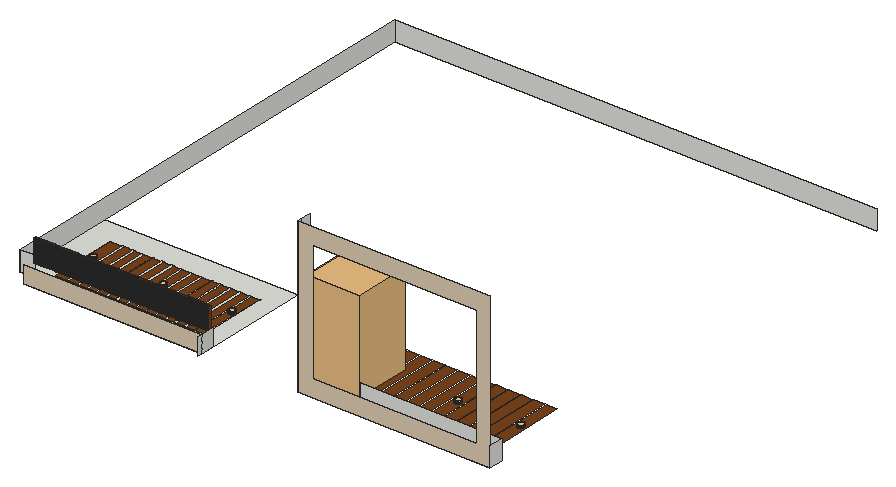
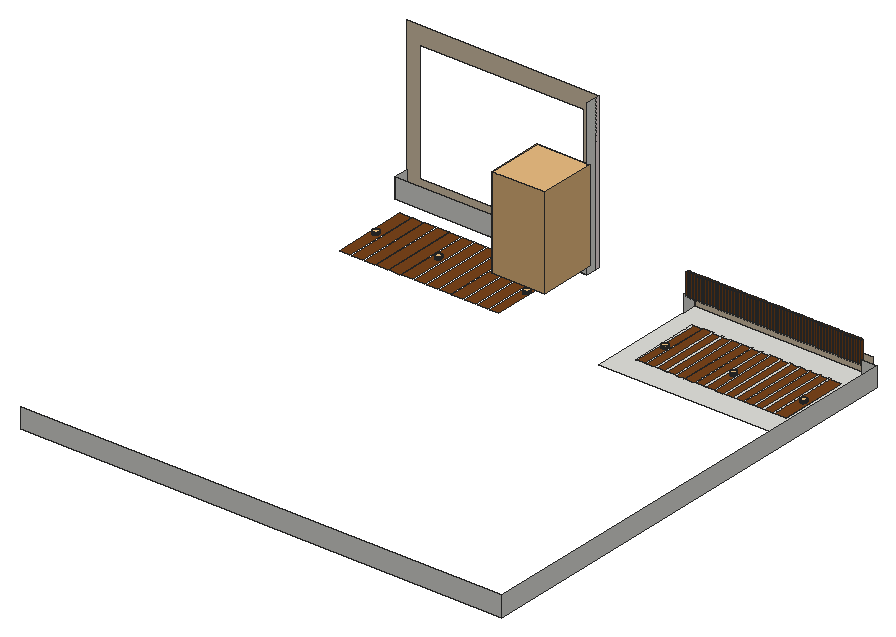
# SketchUp Ruby script. Lengths in inches.
U = 1.inch
M = Sketchup.active_model
def pt(a) = Geom::Point3d.new(a.map { |v| v * U })
def face(e, loops, mat)
  f = e.add_face(loops[0].map { |a| pt(a) })
  loops[1..].each { |l| e.add_face(l.map { |a| pt(a) }).erase! }
  f.material = f.back_material = mat if mat
  f
end
# faces: each face lists its corners as indices into pts; further lists are holes
def faces(e, pts, list, mat = nil) = list.each { |f| face(e, (f[0].is_a?(Array) ? f : [f]).map { |l| l.map { |i| pts[i] } }, mat) }
# xy, xz, yz: faces in a plane at the given z, y or x. An outline is a flat list of corners, or four numbers for a rectangle; further outlines are holes
def ring(l) = l.size == 4 ? [[l[0], l[1]], [l[2], l[1]], [l[2], l[3]], [l[0], l[3]]] : l.each_slice(2).to_a
def flat(e, list, mat, &to3) = list.each { |f| face(e, (f[0].is_a?(Array) ? f : [f]).map { |l| ring(l).map { |u, v| to3.(u, v) } }, mat) }
def xy(e, z, list, mat = nil) = flat(e, list, mat) { |x, y| [x, y, z] }
def xz(e, y, list, mat = nil) = flat(e, list, mat) { |x, z| [x, y, z] }
def yz(e, x, list, mat = nil) = flat(e, list, mat) { |y, z| [x, y, z] }
def lines(e, pts, list) = list.each { |a, b| e.add_line(pt(pts[a]), pt(pts[b])) }
# prism: a flat outline (further loops are holes) pulled along v
def prism(e, loops, v, mat = nil)
  f = face(e, loops, mat); d = Geom::Vector3d.new(v.map { |x| x * U })
  f.pushpull(f.normal.samedirection?(d) ? d.length : -d.length)
end
def box(e, o, s, mat = nil) = prism(e, [[o, [o[0] + s[0], o[1], o[2]], [o[0] + s[0], o[1] + s[1], o[2]], [o[0], o[1] + s[1], o[2]]]], [0, 0, s[2]], mat)
def at(x, y, z, deg = 0) = Geom::Transformation.translation(pt([x, y, z])) * Geom::Transformation.rotation(ORIGIN, Z_AXIS, deg.degrees)
def axes(o, x, y, z) = Geom::Transformation.new([*x, 0, *y, 0, *z, 0, *pt(o).to_a, 1])
def part(name) = M.definitions.add(name)
# library, detail: a bought-in or finely detailed component or shape, given as its bounding box
def library(name, o, s) = part(name).tap { |d| box(d.entities, o, s) }
def detail(e, o, s) = box(e.add_group.entities, o, s)
def put(e, d, t, mat = nil) = e.add_instance(d, t).tap { |i| i.material = mat if mat }
def group(e, t, mat = nil) = e.add_group.tap { |g| g.transformation = t; g.material = mat if mat }.entities
root = M.entities
M.materials.add("Generic\#1").color = [121, 68, 27]
M.materials.add("Generic\#2").color = [245, 199, 133]
M.materials.add("Generic\#6").color = [223, 205, 179]
M.materials.add("Generic\#9").color = [246, 231, 231]
c1 = library("Plante 4",[-1.67,-6.5,0],[37.31,31.95,64.42])
c2 = part("Group\#9")
xy(c2.entities,22.76,[[0,0,2,3]])
xz(c2.entities,0,[[0,0,2,22.76]])
yz(c2.entities,0,[[0,0,3,22.76]])
yz(c2.entities,2,[[0,0,3,22.76]])
xy(root,260.875,[[306.09,39.375,507.875,54.5625],[[17.125,41,204.09,41,204.09,166.1875,2.3125,166.1875,2.3125,54.5625,17.125,54.5625],[27.64,66.32,186.39,140.86]],[40.89,66.32,42.89,140.86],[51.14,66.32,53.14,140.86],[61.39,66.32,63.39,140.86],
  [71.64,66.32,73.64,140.86],[81.89,66.32,83.89,140.86],[92.14,66.32,94.14,140.86],[102.39,66.32,104.39,140.86],[112.64,66.32,114.64,140.86],
  [122.89,66.32,124.89,140.86],[133.14,66.32,135.14,140.86],[143.39,66.32,145.39,140.86],[153.64,66.32,155.64,140.86],[163.89,66.32,165.89,140.86],
  [174.14,66.32,176.14,140.86],[184.39,66.32,186.39,140.86]])
xy(root,260.875,[[[28.83,66.32,40.89,140.86],[34.54,106.62,35.35,106.72,36.11,107.04,36.75,107.53,37.25,108.18,37.5625,108.93,37.67,109.74,37.5625,110.55,37.25,111.3,36.75,111.95,36.11,112.45,35.35,112.76,34.54,112.87,33.74,112.76,32.98,112.45,32.33,111.95,31.84,111.3,31.53,110.55,31.42,109.74,31.53,108.93,31.84,108.18,32.33,107.53,32.98,107.04,33.74,106.72]],[42.89,66.32,51.14,140.86],[53.14,66.32,61.39,140.86],[63.39,66.32,71.64,140.86],[73.64,66.32,81.89,140.86],
  [83.89,66.32,92.14,140.86],[94.14,66.32,102.39,140.86],[[104.39,66.32,112.64,140.86],[108.29,106.62,109.1,106.72,109.86,107.04,110.5,107.53,111,108.18,111.3125,108.93,111.42,109.74,111.3125,110.55,111,111.3,110.5,111.95,109.86,112.45,109.1,112.76,108.29,112.87,107.49,112.76,106.73,112.45,106.08,111.95,105.59,111.3,105.28,110.55,105.17,109.74,105.28,108.93,105.59,108.18,106.08,107.53,106.73,107.04,107.49,106.72]],[114.64,66.32,122.89,140.86],[124.89,66.32,133.14,140.86],
  [135.14,66.32,143.39,140.86],[145.39,66.32,153.64,140.86],[155.64,66.32,163.89,140.86],[165.89,66.32,174.14,140.86],[[176.14,66.32,184.39,140.86],[180.36,106.62,181.17,106.72,181.92,107.04,182.57,107.53,183.0625,108.18,183.375,108.93,183.48,109.74,183.375,110.55,183.0625,111.3,182.57,111.95,181.92,112.45,181.17,112.76,180.36,112.87,179.55,112.76,178.79,112.45,178.15,111.95,177.65,111.3,177.34,110.55,177.23,109.74,177.34,108.93,177.65,108.18,178.15,107.53,178.79,107.04,179.55,106.72]],
  [[322.02,70.49,331.7,150.26],[326.125,105.74,326.97,105.8,327.77,106.08,328.48,106.55,329.03,107.1875,329.41,107.95,329.57,108.78,329.51,109.63,329.24,110.43,328.76,111.14,328.125,111.69,327.36,112.07,326.53,112.23,325.68,112.17,324.88,111.9,324.18,111.42,323.62,110.78,323.25,110.02,323.08,109.1875,323.14,108.34,323.42,107.54,323.89,106.84,324.53,106.28,325.29,105.91]],[333.7,70.49,344.89,150.26],[346.89,70.49,358.07,150.26],[360.07,70.49,371.26,150.26],[373.26,70.49,384.45,150.26],
  [386.45,70.49,397.64,150.26],[399.64,70.49,410.82,150.26],[[412.82,70.49,424.01,150.26],[418.4375,105.74,419.28,105.8,420.08,106.08,420.79,106.55,421.35,107.1875,421.72,107.95,421.88,108.78,421.82,109.63,421.55,110.43,421.08,111.14,420.4375,111.69,419.67,112.07,418.84,112.23,417.99,112.17,417.19,111.9,416.49,111.42,415.93,110.78,415.56,110.02,415.39,109.1875,415.45,108.34,415.73,107.54,416.2,106.84,416.84,106.28,417.6,105.91]],[426.01,70.49,437.2,150.26],[439.2,70.49,450.39,150.26],
  [452.39,70.49,463.57,150.26],[465.57,70.49,476.76,150.26],[[478.76,70.49,489.95,150.26],[484.375,105.74,485.22,105.8,486.02,106.08,486.73,106.55,487.28,107.1875,487.66,107.95,487.82,108.78,487.76,109.63,487.49,110.43,487.01,111.14,486.375,111.69,485.61,112.07,484.78,112.23,483.93,112.17,483.13,111.9,482.43,111.42,481.87,110.78,481.5,110.02,481.33,109.1875,481.39,108.34,481.67,107.54,482.14,106.84,482.78,106.28,483.54,105.91]]],"Generic\#1")
xy(root,263.4375,[[326.125,105.74,325.29,105.91,324.53,106.28,323.89,106.84,323.42,107.54,323.14,108.34,323.08,109.1875,323.25,110.02,323.62,110.78,324.18,111.42,324.88,111.9,325.68,112.17,326.53,112.23,327.36,112.07,328.125,111.69,328.76,111.14,329.24,110.43,329.51,109.63,329.57,108.78,329.41,107.95,329.03,107.1875,328.48,106.55,327.77,106.08,326.97,105.8],[418.4375,105.74,417.6,105.91,416.84,106.28,416.2,106.84,415.73,107.54,415.45,108.34,415.39,109.1875,415.56,110.02,415.93,110.78,416.49,111.42,417.19,111.9,417.99,112.17,418.84,112.23,419.67,112.07,420.4375,111.69,421.08,111.14,421.55,110.43,421.82,109.63,421.88,108.78,421.72,107.95,421.35,107.1875,420.79,106.55,420.08,106.08,419.28,105.8],[484.375,105.74,483.54,105.91,482.78,106.28,482.14,106.84,481.67,107.54,481.39,108.34,481.33,109.1875,481.5,110.02,481.87,110.78,482.43,111.42,483.13,111.9,483.93,112.17,484.78,112.23,485.61,112.07,486.375,111.69,487.01,111.14,487.49,110.43,487.76,109.63,487.82,108.78,487.66,107.95,487.28,107.1875,486.73,106.55,486.02,106.08,485.22,105.8],[34.54,106.62,33.74,106.72,32.98,107.04,32.33,107.53,31.84,108.18,31.53,108.93,31.42,109.74,31.53,110.55,31.84,111.3,32.33,111.95,32.98,112.45,33.74,112.76,34.54,112.87,35.35,112.76,36.11,112.45,36.75,111.95,37.25,111.3,37.5625,110.55,37.67,109.74,37.5625,108.93,37.25,108.18,36.75,107.53,36.11,107.04,35.35,106.72],[108.29,106.62,107.49,106.72,106.73,107.04,106.08,107.53,105.59,108.18,105.28,108.93,105.17,109.74,105.28,110.55,105.59,111.3,106.08,111.95,106.73,112.45,107.49,112.76,108.29,112.87,109.1,112.76,109.86,112.45,110.5,111.95,111,111.3,111.3125,110.55,111.42,109.74,111.3125,108.93,111,108.18,110.5,107.53,109.86,107.04,109.1,106.72],
  [180.36,106.62,179.55,106.72,178.79,107.04,178.15,107.53,177.65,108.18,177.34,108.93,177.23,109.74,177.34,110.55,177.65,111.3,178.15,111.95,178.79,112.45,179.55,112.76,180.36,112.87,181.17,112.76,181.92,112.45,182.57,111.95,183.0625,111.3,183.375,110.55,183.48,109.74,183.375,108.93,183.0625,108.18,182.57,107.53,181.92,107.04,181.17,106.72]],"Generic\#2")
xz(root,39.375,[[[306.09,260.875,507.875,422.625],[321.31,278.625,494.1875,404.6875]]],"Generic\#6")
xz(root,41,[[17.125,260.875,204.09,278.75]],"Generic\#6")
xz(root,54.5625,[[2.3125,260.875,17.125,281.75],[306.09,260.875,507.875,281.75]])
xz(root,546.8125,[[2.3125,260.875,507.875,281.75]])
yz(root,2.3125,[[54.5625,260.875,546.8125,281.75]])
yz(root,204.09,[[35.5625,260.875,41,278.75],[41,260.875,54.5625,278.75]])
yz(root,306.09,[[43.625,260.875,54.5625,422.625]])
yz(root,306.09,[[39.375,260.875,43.625,422.625]],"Generic\#9")
yz(root,507.875,[[39.375,260.875,54.5625,281.75]])
p = [[326.125,105.74,260.875],[325.29,105.91,260.875],[325.29,105.91,263.4375],[326.125,105.74,263.4375],[326.97,105.8,260.875],[326.97,105.8,263.4375],
  [418.4375,105.74,260.875],[417.6,105.91,260.875],[417.6,105.91,263.4375],[418.4375,105.74,263.4375],[419.28,105.8,260.875],[419.28,105.8,263.4375],
  [484.375,105.74,260.875],[483.54,105.91,260.875],[483.54,105.91,263.4375],[484.375,105.74,263.4375],[485.22,105.8,260.875],[485.22,105.8,263.4375],
  [327.77,106.08,260.875],[327.77,106.08,263.4375],[420.08,106.08,260.875],[420.08,106.08,263.4375],[486.02,106.08,260.875],[486.02,106.08,263.4375],
  [324.53,106.28,260.875],[324.53,106.28,263.4375],[416.84,106.28,260.875],[416.84,106.28,263.4375],[482.78,106.28,260.875],[482.78,106.28,263.4375],
  [328.48,106.55,260.875],[328.48,106.55,263.4375],[420.79,106.55,260.875],[420.79,106.55,263.4375],[486.73,106.55,260.875],[486.73,106.55,263.4375],
  [323.89,106.84,260.875],[323.89,106.84,263.4375],[416.2,106.84,260.875],[416.2,106.84,263.4375],[482.14,106.84,260.875],[482.14,106.84,263.4375],
  [329.03,107.1875,260.875],[329.03,107.1875,263.4375],[421.35,107.1875,260.875],[421.35,107.1875,263.4375],[487.28,107.1875,260.875],[487.28,107.1875,263.4375],
  [34.54,106.62,260.875],[33.74,106.72,260.875],[33.74,106.72,263.4375],[34.54,106.62,263.4375],[35.35,106.72,260.875],[35.35,106.72,263.4375],
  [108.29,106.62,260.875],[107.49,106.72,260.875],[107.49,106.72,263.4375],[108.29,106.62,263.4375],[109.1,106.72,260.875],[109.1,106.72,263.4375],
  [180.36,106.62,260.875],[179.55,106.72,260.875],[179.55,106.72,263.4375],[180.36,106.62,263.4375],[181.17,106.72,260.875],[181.17,106.72,263.4375],
  [32.98,107.04,260.875],[32.98,107.04,263.4375],[36.11,107.04,260.875],[36.11,107.04,263.4375],[106.73,107.04,260.875],[106.73,107.04,263.4375],
  [109.86,107.04,260.875],[109.86,107.04,263.4375],[178.79,107.04,260.875],[178.79,107.04,263.4375],[181.92,107.04,260.875],[181.92,107.04,263.4375],
  [323.42,107.54,260.875],[323.42,107.54,263.4375],[415.73,107.54,260.875],[415.73,107.54,263.4375],[481.67,107.54,260.875],[481.67,107.54,263.4375],
  [32.33,107.53,260.875],[32.33,107.53,263.4375],[36.75,107.53,260.875],[36.75,107.53,263.4375],[106.08,107.53,260.875],[106.08,107.53,263.4375],
  [110.5,107.53,260.875],[110.5,107.53,263.4375],[178.15,107.53,260.875],[178.15,107.53,263.4375],[182.57,107.53,260.875],[182.57,107.53,263.4375],
  [329.41,107.95,260.875],[329.41,107.95,263.4375],[421.72,107.95,260.875],[421.72,107.95,263.4375],[487.66,107.95,260.875],[487.66,107.95,263.4375],
  [31.84,108.18,260.875],[31.84,108.18,263.4375],[37.25,108.18,260.875],[37.25,108.18,263.4375],[105.59,108.18,260.875],[105.59,108.18,263.4375],
  [111,108.18,260.875],[111,108.18,263.4375],[177.65,108.18,260.875],[177.65,108.18,263.4375],[183.0625,108.18,260.875],[183.0625,108.18,263.4375],
  [323.14,108.34,260.875],[323.14,108.34,263.4375],[415.45,108.34,260.875],[415.45,108.34,263.4375],[481.39,108.34,260.875],[481.39,108.34,263.4375],
  [329.57,108.78,260.875],[329.57,108.78,263.4375],[421.88,108.78,260.875],[421.88,108.78,263.4375],[487.82,108.78,260.875],[487.82,108.78,263.4375],
  [31.53,108.93,260.875],[31.53,108.93,263.4375],[37.5625,108.93,260.875],[37.5625,108.93,263.4375],[105.28,108.93,260.875],[105.28,108.93,263.4375],
  [111.3125,108.93,260.875],[111.3125,108.93,263.4375],[177.34,108.93,260.875],[177.34,108.93,263.4375],[183.375,108.93,260.875],[183.375,108.93,263.4375],
  [323.08,109.1875,260.875],[323.08,109.1875,263.4375],[415.39,109.1875,260.875],[415.39,109.1875,263.4375],[481.33,109.1875,260.875],[481.33,109.1875,263.4375],
  [329.51,109.63,260.875],[329.51,109.63,263.4375],[421.82,109.63,260.875],[421.82,109.63,263.4375],[487.76,109.63,260.875],[487.76,109.63,263.4375],
  [31.42,109.74,260.875],[31.42,109.74,263.4375],[37.67,109.74,260.875],[37.67,109.74,263.4375],[105.17,109.74,260.875],[105.17,109.74,263.4375],
  [111.42,109.74,260.875],[111.42,109.74,263.4375],[177.23,109.74,260.875],[177.23,109.74,263.4375],[183.48,109.74,260.875],[183.48,109.74,263.4375],
  [323.25,110.02,260.875],[323.25,110.02,263.4375],[415.56,110.02,260.875],[415.56,110.02,263.4375],[481.5,110.02,260.875],[481.5,110.02,263.4375],
  [329.24,110.43,260.875],[329.24,110.43,263.4375],[421.55,110.43,260.875],[421.55,110.43,263.4375],[487.49,110.43,260.875],[487.49,110.43,263.4375],
  [31.53,110.55,260.875],[31.53,110.55,263.4375],[37.5625,110.55,260.875],[37.5625,110.55,263.4375],[105.28,110.55,260.875],[105.28,110.55,263.4375],
  [111.3125,110.55,260.875],[111.3125,110.55,263.4375],[177.34,110.55,260.875],[177.34,110.55,263.4375],[183.375,110.55,260.875],[183.375,110.55,263.4375],
  [323.62,110.78,260.875],[323.62,110.78,263.4375],[415.93,110.78,260.875],[415.93,110.78,263.4375],[481.87,110.78,260.875],[481.87,110.78,263.4375],
  [328.76,111.14,260.875],[328.76,111.14,263.4375],[421.08,111.14,260.875],[421.08,111.14,263.4375],[487.01,111.14,260.875],[487.01,111.14,263.4375],
  [31.84,111.3,260.875],[31.84,111.3,263.4375],[37.25,111.3,260.875],[37.25,111.3,263.4375],[105.59,111.3,260.875],[105.59,111.3,263.4375],
  [111,111.3,260.875],[111,111.3,263.4375],[177.65,111.3,260.875],[177.65,111.3,263.4375],[183.0625,111.3,260.875],[183.0625,111.3,263.4375],
  [324.18,111.42,260.875],[324.18,111.42,263.4375],[416.49,111.42,260.875],[416.49,111.42,263.4375],[482.43,111.42,260.875],[482.43,111.42,263.4375],
  [328.125,111.69,260.875],[328.125,111.69,263.4375],[420.4375,111.69,260.875],[420.4375,111.69,263.4375],[486.375,111.69,260.875],[486.375,111.69,263.4375],
  [32.33,111.95,260.875],[32.33,111.95,263.4375],[36.75,111.95,260.875],[36.75,111.95,263.4375],[106.08,111.95,260.875],[106.08,111.95,263.4375],
  [110.5,111.95,260.875],[110.5,111.95,263.4375],[178.15,111.95,260.875],[178.15,111.95,263.4375],[182.57,111.95,260.875],[182.57,111.95,263.4375],
  [324.88,111.9,260.875],[324.88,111.9,263.4375],[417.19,111.9,260.875],[417.19,111.9,263.4375],[483.13,111.9,260.875],[483.13,111.9,263.4375],
  [327.36,112.07,260.875],[327.36,112.07,263.4375],[419.67,112.07,260.875],[419.67,112.07,263.4375],[485.61,112.07,260.875],[485.61,112.07,263.4375],
  [325.68,112.17,260.875],[325.68,112.17,263.4375],[417.99,112.17,260.875],[417.99,112.17,263.4375],[483.93,112.17,260.875],[483.93,112.17,263.4375],
  [32.98,112.45,260.875],[32.98,112.45,263.4375],[36.11,112.45,260.875],[36.11,112.45,263.4375],[106.73,112.45,260.875],[106.73,112.45,263.4375],
  [109.86,112.45,260.875],[109.86,112.45,263.4375],[178.79,112.45,260.875],[178.79,112.45,263.4375],[181.92,112.45,260.875],[181.92,112.45,263.4375],
  [326.53,112.23,260.875],[326.53,112.23,263.4375],[418.84,112.23,260.875],[418.84,112.23,263.4375],[484.78,112.23,260.875],[484.78,112.23,263.4375],
  [33.74,112.76,260.875],[33.74,112.76,263.4375],[35.35,112.76,260.875],[35.35,112.76,263.4375],[107.49,112.76,260.875],[107.49,112.76,263.4375],
  [109.1,112.76,260.875],[109.1,112.76,263.4375],[179.55,112.76,260.875],[179.55,112.76,263.4375],[181.17,112.76,260.875],[181.17,112.76,263.4375],
  [34.54,112.87,260.875],[34.54,112.87,263.4375],[108.29,112.87,260.875],[108.29,112.87,263.4375],[180.36,112.87,260.875],[180.36,112.87,263.4375]]
faces(root,p,[[0,1,2,3],[4,0,3,5],[6,7,8,9],[10,6,9,11],[12,13,14,15],[16,12,15,17],[18,4,5,19],[20,10,11,21],
  [22,16,17,23],[1,24,25,2],[7,26,27,8],[13,28,29,14],[30,18,19,31],[32,20,21,33],[34,22,23,35],[24,36,37,25],
  [26,38,39,27],[28,40,41,29],[42,30,31,43],[44,32,33,45],[46,34,35,47],[48,49,50,51],[52,48,51,53],[54,55,56,57],
  [58,54,57,59],[60,61,62,63],[64,60,63,65],[49,66,67,50],[68,52,53,69],[55,70,71,56],[72,58,59,73],[61,74,75,62],
  [76,64,65,77],[36,78,79,37],[38,80,81,39],[40,82,83,41],[66,84,85,67],[86,68,69,87],[70,88,89,71],[90,72,73,91],
  [74,92,93,75],[94,76,77,95],[96,42,43,97],[98,44,45,99],[100,46,47,101],[84,102,103,85],[104,86,87,105],[88,106,107,89],
  [108,90,91,109],[92,110,111,93],[112,94,95,113],[78,114,115,79],[80,116,117,81],[82,118,119,83],[120,96,97,121],[122,98,99,123],
  [124,100,101,125],[102,126,127,103],[128,104,105,129],[106,130,131,107],[132,108,109,133],[110,134,135,111],[136,112,113,137],[114,138,139,115],
  [116,140,141,117],[118,142,143,119],[144,120,121,145],[146,122,123,147],[148,124,125,149],[126,150,151,127],[152,128,129,153],[130,154,155,131],
  [156,132,133,157],[134,158,159,135],[160,136,137,161],[138,162,163,139],[140,164,165,141],[142,166,167,143],[168,144,145,169],[170,146,147,171],
  [172,148,149,173],[150,174,175,151],[176,152,153,177],[154,178,179,155],[180,156,157,181],[158,182,183,159],[184,160,161,185],[162,186,187,163],
  [164,188,189,165],[166,190,191,167],[192,168,169,193],[194,170,171,195],[196,172,173,197],[174,198,199,175],[200,176,177,201],[178,202,203,179],
  [204,180,181,205],[182,206,207,183],[208,184,185,209],[186,210,211,187],[188,212,213,189],[190,214,215,191],[216,192,193,217],[218,194,195,219],
  [220,196,197,221],[198,222,223,199],[224,200,201,225],[202,226,227,203],[228,204,205,229],[206,230,231,207],[232,208,209,233],[210,234,235,211],
  [212,236,237,213],[214,238,239,215],[240,216,217,241],[242,218,219,243],[244,220,221,245],[234,246,247,235],[236,248,249,237],[238,250,251,239],
  [222,252,253,223],[254,224,225,255],[226,256,257,227],[258,228,229,259],[230,260,261,231],[262,232,233,263],[264,240,241,265],[266,242,243,267],
  [268,244,245,269],[246,264,265,247],[248,266,267,249],[250,268,269,251],[252,270,271,253],[272,254,255,273],[256,274,275,257],[276,258,259,277],
  [260,278,279,261],[280,262,263,281],[270,282,283,271],[282,272,273,283],[274,284,285,275],[284,276,277,285],[278,286,287,279],[286,280,281,287]],"Generic\#2")
put(root,c1,axes([306.59,65.4375,268.84],[1.4848,0,0],[0,1.856,0],[0,0,1.4848]))
put(root,c2,at(18.375,51.5625,276.75),"Generic\#1")
put(root,c2,at(21.375,51.5625,276.75),"Generic\#1")
put(root,c2,at(24.375,51.5625,276.75),"Generic\#1")
put(root,c2,at(27.375,51.5625,276.75),"Generic\#1")
put(root,c2,at(30.375,51.5625,276.75),"Generic\#1")
put(root,c2,at(33.375,51.5625,276.75),"Generic\#1")
put(root,c2,at(36.375,51.5625,276.75),"Generic\#1")
put(root,c2,at(39.375,51.5625,276.75),"Generic\#1")
put(root,c2,at(42.375,51.5625,276.75),"Generic\#1")
put(root,c2,at(45.375,51.5625,276.75),"Generic\#1")
put(root,c2,at(48.375,51.5625,276.75),"Generic\#1")
put(root,c2,at(51.375,51.5625,276.75),"Generic\#1")
put(root,c2,at(54.375,51.5625,276.75),"Generic\#1")
put(root,c2,at(57.375,51.5625,276.75),"Generic\#1")
put(root,c2,at(60.375,51.5625,276.75),"Generic\#1")
put(root,c2,at(63.375,51.5625,276.75),"Generic\#1")
put(root,c2,at(66.375,51.5625,276.75),"Generic\#1")
put(root,c2,at(69.375,51.5625,276.75),"Generic\#1")
put(root,c2,at(72.375,51.5625,276.75),"Generic\#1")
put(root,c2,at(75.375,51.5625,276.75),"Generic\#1")
put(root,c2,at(78.375,51.5625,276.75),"Generic\#1")
put(root,c2,at(81.375,51.5625,276.75),"Generic\#1")
put(root,c2,at(84.375,51.5625,276.75),"Generic\#1")
put(root,c2,at(87.375,51.5625,276.75),"Generic\#1")
put(root,c2,at(90.375,51.5625,276.75),"Generic\#1")
put(root,c2,at(93.375,51.5625,276.75),"Generic\#1")
put(root,c2,at(96.375,51.5625,276.75),"Generic\#1")
put(root,c2,at(99.375,51.5625,276.75),"Generic\#1")
put(root,c2,at(102.375,51.5625,276.75),"Generic\#1")
put(root,c2,at(105.375,51.5625,276.75),"Generic\#1")
put(root,c2,at(108.375,51.5625,276.75),"Generic\#1")
put(root,c2,at(111.375,51.5625,276.75),"Generic\#1")
put(root,c2,at(114.375,51.5625,276.75),"Generic\#1")
put(root,c2,at(117.375,51.5625,276.75),"Generic\#1")
put(root,c2,at(120.375,51.5625,276.75),"Generic\#1")
put(root,c2,at(123.375,51.5625,276.75),"Generic\#1")
put(root,c2,at(126.375,51.5625,276.75),"Generic\#1")
put(root,c2,at(129.375,51.5625,276.75),"Generic\#1")
put(root,c2,at(132.375,51.5625,276.75),"Generic\#1")
put(root,c2,at(135.375,51.5625,276.75),"Generic\#1")
put(root,c2,at(138.375,51.5625,276.75),"Generic\#1")
put(root,c2,at(141.375,51.5625,276.75),"Generic\#1")
put(root,c2,at(144.375,51.5625,276.75),"Generic\#1")
put(root,c2,at(147.375,51.5625,276.75),"Generic\#1")
put(root,c2,at(150.375,51.5625,276.75),"Generic\#1")
put(root,c2,at(153.375,51.5625,276.75),"Generic\#1")
put(root,c2,at(156.375,51.5625,276.75),"Generic\#1")
put(root,c2,at(159.375,51.5625,276.75),"Generic\#1")
put(root,c2,at(162.375,51.5625,276.75),"Generic\#1")
put(root,c2,at(165.375,51.5625,276.75),"Generic\#1")
put(root,c2,at(168.375,51.5625,276.75),"Generic\#1")
put(root,c2,at(171.3125,51.5625,276.75),"Generic\#1")
put(root,c2,at(174.25,51.5625,276.75),"Generic\#1")
put(root,c2,at(177.1875,51.5625,276.75),"Generic\#1")
put(root,c2,at(180.125,51.5625,276.75),"Generic\#1")
put(root,c2,at(183.0625,51.5625,276.75),"Generic\#1")
put(root,c2,at(186,51.5625,276.75),"Generic\#1")
put(root,c2,at(188.9375,51.5625,276.75),"Generic\#1")
put(root,c2,at(191.875,51.5625,276.75),"Generic\#1")
put(root,c2,at(194.8125,51.5625,276.75),"Generic\#1")
put(root,c2,at(197.75,51.5625,276.75),"Generic\#1")
put(root,c2,at(200.8125,51.5625,276.75),"Generic\#1")
